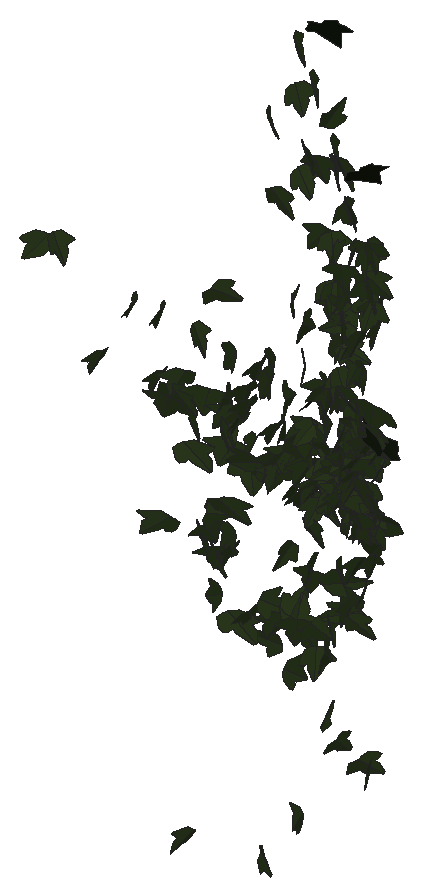
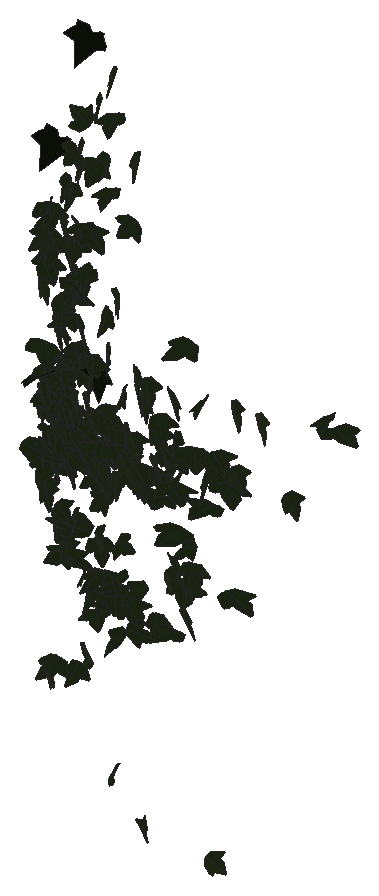
# SketchUp Ruby script. Lengths in millimetres.
U = 1.mm
M = Sketchup.active_model
def pt(a) = Geom::Point3d.new(a.map { |v| v * U })
def face(e, loops, mat)
  f = e.add_face(loops[0].map { |a| pt(a) })
  loops[1..].each { |l| e.add_face(l.map { |a| pt(a) }).erase! }
  f.material = f.back_material = mat if mat
  f
end
# faces: each face lists its corners as indices into pts; further lists are holes
def faces(e, pts, list, mat = nil) = list.each { |f| face(e, (f[0].is_a?(Array) ? f : [f]).map { |l| l.map { |i| pts[i] } }, mat) }
# xy, xz, yz: faces in a plane at the given z, y or x. An outline is a flat list of corners, or four numbers for a rectangle; further outlines are holes
def ring(l) = l.size == 4 ? [[l[0], l[1]], [l[2], l[1]], [l[2], l[3]], [l[0], l[3]]] : l.each_slice(2).to_a
def flat(e, list, mat, &to3) = list.each { |f| face(e, (f[0].is_a?(Array) ? f : [f]).map { |l| ring(l).map { |u, v| to3.(u, v) } }, mat) }
def xy(e, z, list, mat = nil) = flat(e, list, mat) { |x, y| [x, y, z] }
def xz(e, y, list, mat = nil) = flat(e, list, mat) { |x, z| [x, y, z] }
def yz(e, x, list, mat = nil) = flat(e, list, mat) { |y, z| [x, y, z] }
def lines(e, pts, list) = list.each { |a, b| e.add_line(pt(pts[a]), pt(pts[b])) }
# prism: a flat outline (further loops are holes) pulled along v
def prism(e, loops, v, mat = nil)
  f = face(e, loops, mat); d = Geom::Vector3d.new(v.map { |x| x * U })
  f.pushpull(f.normal.samedirection?(d) ? d.length : -d.length)
end
def box(e, o, s, mat = nil) = prism(e, [[o, [o[0] + s[0], o[1], o[2]], [o[0] + s[0], o[1] + s[1], o[2]], [o[0], o[1] + s[1], o[2]]]], [0, 0, s[2]], mat)
def at(x, y, z, deg = 0) = Geom::Transformation.translation(pt([x, y, z])) * Geom::Transformation.rotation(ORIGIN, Z_AXIS, deg.degrees)
def axes(o, x, y, z) = Geom::Transformation.new([*x, 0, *y, 0, *z, 0, *pt(o).to_a, 1])
def part(name) = M.definitions.add(name)
# library, detail: a bought-in or finely detailed component or shape, given as its bounding box
def library(name, o, s) = part(name).tap { |d| box(d.entities, o, s) }
def detail(e, o, s) = box(e.add_group.entities, o, s)
def put(e, d, t, mat = nil) = e.add_instance(d, t).tap { |i| i.material = mat if mat }
def group(e, t, mat = nil) = e.add_group.tap { |g| g.transformation = t; g.material = mat if mat }.entities
root = M.entities
M.materials.add("efeu1").color = [18, 25, 13]
M.materials.add("efeu2").color = [43, 57, 29]
c1 = part("ivyleaf_10")
p = [[0,12.8,-0.8],[-1.5,51.3,-10.9],[-4.9,51,-11.6],[-13.6,26.5,-7.3],[-13.2,15.9,-4.6],[-21.1,19.3,-7.2],
  [-29.5,16.3,-8.3],[-29.2,8.3,-6.2],[-19.7,-9.8,0.5],[-7.6,-13,4],[1,-12.2,5.8],[-0.4,51.1,-11.1],
  [-1.5,51.1,-10.9],[1,-12.4,5.9],[16.9,-12.4,3.5],[35.1,9.1,-5.1],[35,12.9,-6.1],[20.5,16.4,-4.9],
  [15.8,15,-3.8],[15.3,27.6,-7.1],[12.8,31.3,-7.8]]
faces(c1.entities,p,[[0,1,2,3,4,5,6,7,8,9,10],[11,12,0,13,14,15,16,17,18,19,20]],"efeu2")
c2 = part("ivyleaf_9")
p = [[39.1,54.8,31.7],[34.5,51.8,30.2],[-5.3,25.2,17.3],[-17.9,28.3,20.9],[-21.6,21.7,17],[-20.2,4.3,5.3],
  [-22.9,-0.3,2.5],[-17.1,-4,-0.6],[-2,-2.1,-1.2],[-0.7,-15.4,-10.1],[16.6,-22.3,-16.7],[21.1,-15.1,-12.5],
  [32.7,-10.7,-11],[46.1,-1.8,-6.6],[30.8,11.2,3.8]]
faces(c2.entities,p,[[0,1,2,3,4,5,6,7,8,9,10,11,12,13,14]],"efeu1")
put(root,c1,axes([280.1,1052.8,968.5],[0.80432,0.38706,-0.36071],[-0.57294,-0.20372,-0.57131],[-0.82806,0.51692,0.04493]))
put(root,c1,axes([304.2,1049,979.4],[0.14498,0.67726,0.04064],[-0.0098,0.04147,-0.68146],[-1.29124,0.07573,0.00973]))
put(root,c1,axes([369.6,1059.6,820.7],[-0.10799,-0.6367,0.11101],[0.00127,-0.1115,-0.63914],[1.23005,-0.05578,0.01041]))
put(root,c1,axes([435.9,1048.1,929.1],[0.18821,-0.63502,-0.20371],[-0.07183,0.20028,-0.64264],[1.2672,0.10567,-0.00617]))
put(root,c1,axes([474.4,1058,828.7],[-0.07826,-0.64651,0.07347],[-0.00557,-0.07344,-0.64781],[1.23834,-0.04119,0.00173]))
put(root,c1,axes([485.9,1053.1,609.2],[-0.72644,-0.3296,0.38813],[-0.44742,-0.31621,-0.49971],[0.85963,-0.44311,0.0679]))
put(root,c1,axes([484.6,1047.2,933.6],[0.18486,-0.65896,-0.1229],[0.01618,0.12538,-0.66557],[1.27566,0.0939,0.02625]))
put(root,c1,axes([496.1,1051,796.7],[-1.17512,-0.07231,0.17501],[-0.33467,-0.00247,-0.62142],[0.13369,-0.64176,-0.01733]))
put(root,c1,axes([514.7,1056,841],[-0.50585,-0.5574,0.22476],[-0.00833,-0.24396,-0.61018],[1.14381,-0.24829,0.09496]))
put(root,c1,axes([507.6,1049.3,818.6],[-1.10365,0.06979,-0.28827],[0.53343,-0.07811,-0.58274],[-0.18462,-0.64286,0.03951]))
put(root,c1,axes([524.9,1054.5,138.6],[-0.02119,-0.50512,0.39183],[-0.00233,-0.39187,-0.50521],[1.21668,-0.00955,0.00586]))
put(root,c1,axes([543.1,1043.6,782.1],[-0.43934,0.51009,0.32121],[-0.30419,0.27986,-0.55928],[-1.10619,-0.27955,0.02622]))
put(root,c1,axes([546,1048.1,923.3],[-0.06976,0.6764,0.00446],[-0.00032,0.00445,-0.67739],[-1.28735,-0.03666,-0.00007]))
put(root,c1,axes([537.8,1041.8,741.6],[0.76421,0.35078,0.36417],[0.45923,0.27573,-0.53165],[-0.84568,0.46672,0.04039]))
put(root,c1,axes([561.3,1049.4,597.1],[-0.64382,0.54486,-0.11963],[-0.12189,0.10105,0.64133],[1.05466,0.34429,0.00109]))
put(root,c1,axes([561.7,1053.1,830.7],[-1.06464,-0.33047,0.09999],[-0.02614,-0.16892,-0.63514],[0.65658,-0.54257,0.13684]))
put(root,c1,axes([565.4,1050,628.1],[-0.52647,-0.55222,-0.22368],[0.22261,0.19147,-0.61738],[1.11186,-0.29982,0.0177]))
put(root,c1,axes([579.5,1053.7,594.6],[-0.80133,-0.49881,-0.03379],[0.04217,0.02551,-0.65276],[0.95058,-0.42162,0.00047]))
put(root,c1,axes([585.6,1042.1,535],[0.38899,-0.41925,-0.46224],[-0.40776,0.4097,-0.46633],[1.1155,0.29596,-0.00927]))
put(root,c1,axes([576.9,1038.2,658.1],[-0.0198,-0.29068,-0.5946],[0.48061,0.54794,-0.27229],[1.16433,-0.23112,0.10228]))
put(root,c1,axes([568,1056.1,585.7],[0.19112,-0.21579,0.59118],[0.95073,-0.33678,-0.20779],[0.72848,0.49614,0.11608]))
put(root,c1,axes([584.2,1058,786.8],[-0.13485,0.63887,-0.1144],[0.00021,-0.11507,-0.64267],[-1.23525,-0.06977,0.01238]))
put(root,c1,axes([598.3,1057.9,760.7],[-0.98695,-0.29802,0.24077],[-0.1698,-0.30011,-0.56363],[0.70911,-0.48665,0.20014]))
put(root,c1,axes([585,1040.5,1003.5],[-0.47824,-0.34217,-0.55231],[0.64589,0.43584,-0.42442],[1.05443,-0.42217,0.00948]))
put(root,c1,axes([604.9,1055.4,816.3],[-0.64473,-0.45424,0.33849],[-0.32581,-0.29387,-0.56569],[1.02774,-0.37812,0.03301]))
put(root,c1,axes([596.4,1048.6,843.9],[0.13324,-0.56152,-0.34486],[0.16327,0.35162,-0.55511],[1.24347,0.014,0.10984]))
put(root,c1,axes([592.7,1056.8,798.1],[0.04256,0.65463,-0.0365],[-0.00251,-0.03648,-0.65501],[-1.24782,0.0224,0.00007]))
put(root,c1,axes([600.8,1051.3,629],[0.72732,-0.48918,-0.19687],[-0.14187,0.19057,-0.61824],[0.99349,0.38533,0.05584]))
put(root,c1,axes([601.7,1057.8,605.7],[0.10367,-0.62598,0.15616],[0.00987,-0.15628,-0.6283],[1.22784,0.05411,-0.00814]))
put(root,c1,axes([608.1,1045.3,911.5],[0.65528,-0.54496,-0.20928],[-0.10038,0.21293,-0.64125],[1.10647,0.34206,0.06577]))
put(root,c1,axes([596.7,1044.7,677.7],[-1.03918,-0.15423,-0.35911],[0.64836,0.11457,-0.56718],[0.36455,-0.6434,-0.01491]))
put(root,c1,axes([610,1055.9,808.4],[0.22548,-0.64019,-0.09152],[-0.00084,0.09296,-0.65086],[1.2308,0.11734,0.01632]))
put(root,c1,axes([627.8,1050.1,862.8],[-0.37925,-0.6345,-0.1009],[0.02524,0.10155,-0.66482],[1.22249,-0.19893,-0.01758]))
put(root,c1,axes([609.4,1047.8,502.6],[0.85017,0.33533,0.35778],[0.55087,0.21036,-0.55854],[-0.75333,0.53226,-0.00466]))
put(root,c1,axes([629.5,1052.7,840.4],[-0.24515,-0.65142,-0.05506],[0.01019,0.05506,-0.66401],[1.24416,-0.12881,-0.00541]))
put(root,c1,axes([632.8,1051.8,517.3],[-0.31182,-0.56641,-0.24556],[0.10948,0.23895,-0.58954],[1.16983,-0.17334,-0.01028]))
put(root,c1,axes([646.4,1042.4,758.3],[0.77283,-0.02268,-0.50401],[-0.84507,0.29111,-0.37084],[0.45589,0.57807,0.16698]))
put(root,c1,axes([638.8,1049.9,784.5],[0.53287,-0.61772,0.01758],[0.01416,-0.01592,-0.67821],[1.17604,0.28008,0.0002]))
put(root,c1,axes([628.3,1056.6,736.7],[1.22814,-0.01167,0.17544],[0.33338,-0.01503,-0.64531],[0.02894,0.66856,-0.01145]))
put(root,c1,axes([655.6,1045.1,912.8],[-0.08785,-0.67224,-0.12382],[0.02034,0.12338,-0.67382],[1.30076,-0.04733,0.00217]))
put(root,c1,axes([660.1,1060.3,750.3],[-0.13337,-0.64013,0.02762],[0.00929,-0.02831,-0.64391],[1.21939,-0.0698,0.00792]))
put(root,c1,axes([673.4,1055.6,485],[0.03445,0.03695,-0.70207],[-0.82529,0.19278,-0.01706],[0.23358,0.67567,0.04326]))
put(root,c1,axes([665.2,1057.9,765.8],[-0.23005,-0.60941,0.17977],[-0.08482,-0.17441,-0.62121],[1.20627,-0.12849,-0.0094]))
put(root,c1,axes([662.6,1048.3,887],[0.7927,-0.51225,-0.15366],[0.01192,0.19942,-0.64783],[1.01775,0.39664,0.12727]))
put(root,c1,axes([649.6,1057.6,145.3],[0.04948,-0.02956,0.63621],[0.9191,-0.41422,-0.03898],[0.79027,0.48359,0.0055]))
put(root,c1,axes([673.5,1056.8,817.2],[-0.11354,-0.65426,-0.02118],[-0.01753,0.0221,-0.65688],[1.24572,-0.05932,-0.01117]))
put(root,c1,axes([672.6,1047,896.4],[0.51298,-0.59828,-0.18198],[-0.00743,0.19655,-0.65196],[1.19013,0.2591,0.07437]))
put(root,c1,axes([678.4,1041.6,1296.1],[-0.54273,0.42017,0.38541],[-0.32115,0.28226,-0.61157],[-0.61702,-0.5165,-0.02069]))
put(root,c1,axes([670.4,1041.8,552],[0.08884,0.38468,0.60598],[0.10993,0.59937,-0.39131],[-0.86874,0.11518,0.01245]))
put(root,c1,axes([683.2,1056.8,525],[-0.56316,-0.56367,0.2269],[-0.14207,-0.21674,-0.63577],[1.14767,-0.30342,0.03264]))
put(root,c1,axes([677.4,1044.8,925.6],[0.58022,-0.55116,-0.27285],[0.00028,0.30461,-0.61513],[1.17046,0.27314,0.13541]))
put(root,c1,axes([682.2,1044.2,748],[0.35069,-0.59688,-0.22796],[-0.0606,0.22837,-0.62371],[1.2145,0.18375,0.0347]))
put(root,c1,axes([684.4,1055.7,752.9],[-0.54362,-0.52681,0.236],[-0.03889,-0.25391,-0.59154],[1.09794,-0.26983,0.0959]))
put(root,c1,axes([687.5,1060.9,776.1],[-0.09249,-0.63599,0.10402],[-0.03026,-0.1031,-0.6378],[1.22613,-0.05052,-0.00789]))
put(root,c1,axes([682.1,1049.1,1181.9],[-0.71162,0.11038,-0.40021],[0.46362,-0.13593,-0.59136],[-0.20393,-0.69421,0.05216]))
put(root,c1,axes([693.1,1063.7,632.4],[0.05493,0.48939,-0.48758],[-0.3037,-0.4443,-0.46893],[-0.78618,0.20582,0.14708]))
put(root,c1,axes([690.8,1052.1,826.1],[0.33863,-0.574,-0.2759],[0.09951,0.29867,-0.58764],[1.20799,0.1363,0.12575]))
put(root,c1,axes([703.5,1057.6,786.3],[-0.94893,-0.37717,0.18792],[-0.11506,-0.22408,-0.61017],[0.7937,-0.48343,0.13621]))
put(root,c1,axes([704.5,1040.5,878.4],[0.17993,-0.25751,-0.64935],[0.0939,0.6561,-0.253],[1.32615,-0.01152,0.10602]))
put(root,c1,axes([707.4,1056.4,737.8],[0.01575,-0.59983,-0.22154],[0.06168,0.22167,-0.59896],[1.21541,-0.00348,0.03327]))
put(root,c1,axes([710.2,1042.6,458.7],[-0.03949,0.42903,0.62238],[-0.11634,0.61565,-0.42935],[-0.91486,-0.09681,0.02773]))
put(root,c1,axes([723.9,1033.1,1033.5],[0.02742,0.1723,0.69331],[-0.78872,0.56687,-0.13226],[-1.10751,-0.39944,0.11136]))
put(root,c1,axes([708.3,1064.8,223.8],[-0.24162,0.01373,0.63664],[0.53678,-0.58081,0.06877],[1.08657,0.28998,0.10759]))
put(root,c1,axes([718.1,1056.9,730.5],[-0.15989,-0.60914,-0.1781],[0.04975,0.17618,-0.6149],[1.20682,-0.08797,0.00175]))
put(root,c1,axes([711,1047.6,552.6],[0.32929,0.4724,-0.5018],[0.29847,0.43814,0.54406],[0.78604,-0.36427,0.00363]))
put(root,c1,axes([720.9,1046.9,533.2],[-0.70789,-0.4564,0.07783],[-0.08124,-0.04122,-0.73818],[0.55898,-0.58398,-0.00872]))
put(root,c1,axes([712.9,1050.7,536.4],[0.7773,0.3037,-0.20744],[0.22867,0.08888,0.70581],[0.38605,-0.66413,-0.00041]))
put(root,c1,axes([720.2,1047.1,1428.5],[-0.42691,0.64337,0.15248],[-0.10326,0.12751,-0.73226],[-0.80002,-0.35978,0.01314]))
put(root,c1,axes([718.4,1048.4,1353.8],[0.39427,0.63237,0.11758],[0.00984,0.12759,-0.70839],[-0.78465,0.31935,0.0502]))
put(root,c1,axes([726.6,1054,825.7],[-0.28175,-0.64309,-0.06517],[0.0151,0.06505,-0.65987],[1.2301,-0.14809,-0.00683]))
put(root,c1,axes([734.6,1056.5,838.5],[-0.35471,-0.34286,0.56571],[-0.45682,-0.42411,-0.44949],[0.66529,-0.47402,-0.00702]))
put(root,c1,axes([730,1054.8,782.5],[-0.38704,-0.59074,0.1892],[-0.0308,-0.19399,-0.62308],[1.18015,-0.1988,0.04579]))
put(root,c1,axes([722.6,1044.6,808.6],[-0.86242,-0.0504,-0.23627],[0.28807,0.01034,-0.70867],[0.06232,-0.74527,0.00614]))
put(root,c1,axes([731,1051.8,778.2],[-0.36019,-0.59193,0.19072],[-0.04387,-0.19254,-0.62046],[1.18278,-0.1874,0.03507]))
put(root,c1,axes([722.6,1051.7,1224.9],[0.29001,0.63936,0.18485],[0.09862,0.16709,-0.68191],[-0.80595,0.25051,-0.01693]))
put(root,c1,axes([736.4,1039.2,940],[0.26272,-0.37261,-0.62387],[-0.20626,0.60714,-0.42098],[0.86221,0.25878,0.08939]))
put(root,c1,axes([734,1053.5,809.9],[0.56083,-0.58013,-0.09412],[-0.04865,0.09253,-0.6504],[1.11748,0.29518,0.01892]))
put(root,c1,axes([739.4,1055.7,613],[-0.77622,-0.16491,0.17004],[-0.20012,-0.04484,-0.65727],[0.20848,-0.65705,0.00218]))
put(root,c1,axes([734.6,1049.1,522.3],[-0.62799,-0.34601,-0.14546],[0.14847,0.0797,-0.62023],[0.43318,-0.52893,0.0017]))
put(root,c1,axes([739.2,1053.1,841.6],[0.50488,0.34265,-0.39183],[-0.36844,-0.24965,-0.53728],[-0.51722,0.51231,0.00025]))
put(root,c1,axes([736.8,1040.1,1004],[0.00355,-0.44298,-0.59748],[0.04866,0.59672,-0.44222],[0.90611,-0.03031,0.02609]))
put(root,c1,axes([734.3,1064.4,630.5],[0.30211,-0.54842,0.35009],[0.20014,-0.30985,-0.60144],[0.76813,0.29643,0.01901]))
put(root,c1,axes([740.8,1061.1,751.4],[-0.13094,-0.63941,0.05428],[-0.00526,-0.05429,-0.64309],[1.22129,-0.06879,0.00305]))
put(root,c1,axes([739.8,1058.6,750.8],[-0.13978,-0.5592,0.29973],[0.05125,-0.30421,-0.56096],[1.20643,-0.05187,0.05856]))
put(root,c1,axes([738.1,1043.2,1270.3],[-0.6488,0.49186,-0.02565],[0.0257,-0.015,-0.72439],[-0.60034,-0.53221,-0.00329]))
put(root,c1,axes([735.4,1054.4,690],[-0.60101,0.25831,-0.34202],[0.37315,-0.15315,-0.55622],[-0.36631,-0.57983,-0.00546]))
put(root,c1,axes([741.4,1054.2,1375.5],[-0.40851,0.64099,-0.09276],[0.00286,-0.10322,-0.72176],[-0.79015,-0.33177,0.04534]))
put(root,c1,axes([759.2,1052.2,824.2],[-0.36195,0.03985,0.59004],[-0.71403,0.07487,-0.29934],[-0.10345,-0.65617,0.00168]))
put(root,c1,axes([748.3,1055.5,723.2],[0.52253,0.49079,-0.25962],[-0.32433,-0.10659,-0.64007],[-0.59469,0.48937,0.12095]))
put(root,c1,axes([744.2,1055.6,492.2],[0.46112,0.62121,-0.07646],[-0.07922,-0.04992,-0.72657],[-0.75948,0.38238,0.02936]))
put(root,c1,axes([758,1057.5,1145.3],[-0.58993,-0.33267,0.38508],[-0.37938,-0.22731,-0.58686],[0.49142,-0.57483,0.00921]))
put(root,c2,axes([760.7,1035.6,899.2],[-0.00587,0.73457,0.24139],[-0.1084,0.23927,-0.72989],[-0.93707,-0.03228,0.08292]))
put(root,c1,axes([754.9,1047.5,1259.2],[-0.84142,-0.11486,-0.10799],[0.12842,0.02523,-0.69914],[0.14318,-0.69763,-0.00751]))
put(root,c1,axes([759,1051.4,886.7],[-0.41703,0.60905,0.1312],[-0.13926,0.08589,-0.69612],[-0.74722,-0.35592,0.05651]))
put(root,c1,axes([763.5,1050.1,914.7],[-0.74307,-0.40011,0.07551],[-0.03063,-0.0987,-0.72552],[0.4958,-0.60575,0.06834]))
put(root,c1,axes([770.9,1063.3,798.6],[-0.46788,-0.23761,0.5026],[-0.36873,-0.42336,-0.43077],[0.56926,-0.46952,0.13407]))
put(root,c1,axes([755.2,1039.1,545.3],[-0.38195,-0.48468,-0.46335],[0.53588,0.37804,-0.51739],[1.15819,-0.33475,0.08659]))
put(root,c1,axes([771.2,1045.9,916.2],[0.42523,-0.36414,-0.55987],[-0.31702,0.50783,-0.49206],[0.75061,0.42077,0.10935]))
put(root,c1,axes([766.7,1043.2,913.9],[-0.22812,-0.67729,-0.21292],[0.05119,0.20925,-0.70248],[0.86465,-0.19107,-0.01459]))
put(root,c1,axes([766.8,1053.8,850.7],[0.49008,-0.59026,-0.16503],[0.0047,0.18,-0.63996],[1.16645,0.24727,0.07191]))
put(root,c1,axes([762,1058.9,775.2],[1.03244,0.35695,-0.02191],[-0.03691,-0.01038,-0.64938],[-0.67963,0.54282,0.00199]))
put(root,c1,axes([768.9,1055.9,901.4],[-0.06,-0.68772,0.24142],[0.07686,-0.24508,-0.68529],[0.88589,-0.02532,0.07581]))
put(root,c1,axes([771.8,1040.4,508],[0.14065,-0.50236,-0.55334],[0.00914,0.56063,-0.50742],[0.91173,0.07188,0.09045]))
put(root,c1,axes([765.2,1057.8,762.4],[-1.07416,0.18765,-0.23674],[0.35067,-0.18371,-0.5849],[-0.45561,-0.58382,0.10796]))
put(root,c1,axes([768.1,1046.4,397.9],[0.51183,-0.56118,0.14321],[-0.11257,0.13045,0.62229],[-1.09651,-0.27534,0.00296]))
put(root,c1,axes([778.1,1063,752.6],[-0.26766,-0.41537,0.46283],[-0.13204,-0.46107,-0.43487],[1.17618,-0.14629,0.05651]))
put(root,c1,axes([781.7,1055.7,791.7],[0.2926,0.24368,-0.61379],[-0.61825,-0.3508,-0.33729],[-0.5166,0.55785,0.05601]))
put(root,c1,axes([768.8,1048.5,1065.6],[0.30232,0.62315,0.07576],[0.03339,0.07065,-0.67062],[-0.76512,0.24931,0.00067]))
put(root,c1,axes([775.5,1054.4,762.8],[0.45695,-0.60033,-0.06449],[-0.0295,0.06325,-0.6465],[1.14875,0.24043,0.00905]))
put(root,c2,axes([770.6,1038.5,1477.1],[0.72465,0.46252,-0.12405],[-0.09978,-0.09676,-0.75237],[-0.57563,0.59902,-0.02574]))
put(root,c1,axes([769.9,1055.3,551.7],[-0.23147,0.57199,-0.22008],[0.10225,-0.20401,-0.60246],[-0.74068,-0.20692,-0.01439]))
put(root,c1,axes([782,1054.5,984],[0.43738,-0.44174,-0.4577],[-0.33525,0.36628,-0.56875],[0.69989,0.4515,0.01359]))
put(root,c1,axes([755.8,1053.9,735.9],[0.52365,-0.17693,0.57143],[1.00572,-0.22289,-0.32345],[0.53356,0.59377,0.04886]))
put(root,c1,axes([771.2,1060.2,1257.1],[-0.4185,0.57342,-0.25785],[0.15052,-0.22662,-0.66812],[-0.75213,-0.36442,0.00976]))
put(root,c1,axes([774.8,1056.2,1286.9],[-0.41042,0.64415,-0.04422],[-0.01748,-0.0573,-0.72565],[-0.78752,-0.33443,0.03915]))
put(root,c1,axes([783.9,1056.8,791.9],[-0.45885,-0.60692,0.05726],[-0.06567,-0.04789,-0.6529],[1.15836,-0.24313,-0.01433]))
put(root,c1,axes([774.7,1071.3,820.4],[-0.04643,-0.05106,-0.69109],[0.05462,-0.69087,0.04858],[-0.84367,-0.04191,0.04118]))
put(root,c1,axes([775.7,1047,1326.6],[-0.09313,-0.65052,0.34299],[0.03292,0.34212,0.65488],[-0.89658,0.08013,-0.01158]))
put(root,c1,axes([776,1050.2,1145.1],[0.46505,0.55348,0.0293],[0.01953,0.02456,-0.67204],[-0.67591,0.38153,0.00075]))
put(root,c1,axes([788.6,1044.2,911.7],[-0.46759,0.54407,0.22852],[-0.41511,0.01888,-0.61563],[-0.58821,-0.44582,0.25281]))
put(root,c1,axes([779.6,1047.4,1068.7],[0.23362,0.62767,-0.13612],[-0.07614,-0.12319,-0.65581],[-0.77985,0.20006,0.02325]))
put(root,c1,axes([787.1,1048.1,1054.3],[-0.53942,-0.50523,0.15799],[-0.12707,-0.1188,-0.67137],[0.63319,-0.45425,-0.00014]))
put(root,c1,axes([786.1,1057.8,748.8],[-0.1284,-0.58687,0.25621],[0.0135,-0.25829,-0.58978],[1.21865,-0.05897,0.03353]))
put(root,c1,axes([792.1,1037.1,1130.2],[0.39412,0.00931,0.61207],[-0.58526,0.43375,0.24659],[-0.4639,-0.53931,0.2089]))
put(root,c1,axes([788.5,1050.7,915.6],[-0.83808,-0.16614,0.01577],[-0.01878,-0.00342,-0.70676],[0.20274,-0.68712,-0.0003]))
put(root,c1,axes([784.3,1054.2,929.9],[0.33263,0.57164,-0.16029],[-0.07054,-0.14998,-0.63322],[-0.72086,0.27845,-0.012]))
put(root,c1,axes([799.7,1051.3,1021.7],[0.33822,0.10228,-0.58345],[-0.69254,-0.13819,-0.29395],[-0.20648,0.63101,0.0302]))
put(root,c1,axes([803.8,1059.7,574.3],[0.75795,0.12397,-0.51768],[-0.96397,-0.11064,-0.41615],[-0.31167,0.6437,0.02817]))
put(root,c1,axes([787.8,1057.8,848.5],[0.40085,-0.56663,0.16094],[0.10927,-0.13409,-0.65493],[0.71028,0.34041,0.00993]))
put(root,c1,axes([793.8,1045.2,641.5],[-0.41165,0.41011,0.36563],[-0.28026,0.28446,-0.53107],[-0.60891,-0.40818,-0.00275]))
put(root,c1,axes([786.6,1053.6,938.5],[0.17346,0.62258,0.06943],[0.02006,0.06746,-0.6386],[-0.76399,0.14312,-0.001]))
put(root,c1,axes([795.3,1046.4,1064.6],[0.48574,-0.4127,-0.34597],[-0.26233,0.27265,-0.57269],[0.60237,0.45153,0.02958]))
put(root,c1,axes([788.8,1047.8,377.4],[-0.33195,-0.43726,-0.4379],[0.28119,0.41238,-0.47062],[1.14369,-0.2283,-0.01139]))
put(root,c1,axes([790.7,1051,1026.8],[-0.46682,0.47354,-0.26209],[0.15698,-0.23218,-0.60736],[-0.64137,-0.40149,0.0421]))
put(root,c1,axes([801.2,1052.7,1043.3],[0.68286,-0.02827,-0.35294],[-0.4301,0.0169,-0.56044],[0.04017,0.66149,-0.00077]))
put(root,c1,axes([799.1,1044.6,1108.4],[-0.76664,-0.25885,0.01291],[-0.01728,0.00048,-0.67959],[0.31572,-0.62852,-0.00584]))
put(root,c1,axes([793.5,1056.4,1025.5],[-0.14503,0.51849,-0.36064],[0.03924,-0.36152,-0.53037],[-0.76953,-0.11615,0.04092]))
put(root,c1,axes([799.1,1051.1,1075.7],[0.55406,-0.49626,-0.11124],[-0.09391,0.08034,-0.6727],[0.61332,0.46062,-0.00251]))
put(root,c1,axes([794.8,1059.5,789.7],[1.21149,-0.12359,-0.02219],[-0.01822,0.06655,-0.64533],[0.23828,0.63346,0.06347]))
put(root,c1,axes([791.9,1055,815.2],[0.25718,-0.47067,0.42743],[0.35397,-0.32947,-0.5059],[0.69019,0.34436,0.10019]))
put(root,c1,axes([795.3,1059.8,794.6],[0.70511,0.52121,-0.09834],[-0.10611,-0.08102,-0.63946],[-1.00387,0.37465,-0.00148]))
put(root,c1,axes([801.3,1058.3,587],[-0.00074,-0.65883,0.16871],[0.00544,-0.16871,-0.65881],[0.82969,0.00052,0.00447]))
put(root,c1,axes([783.9,1044.5,617.1],[-0.31698,-0.21523,0.6372],[0.70347,0.51913,0.27196],[-1.06939,0.40529,-0.00997]))
put(root,c1,axes([813.8,1053.9,885.2],[-0.26048,0.27092,-0.57718],[-0.63608,0.27619,0.3225],[0.44776,0.54995,0.12237]))
put(root,c1,axes([799,1047.8,1202.5],[-0.03337,-0.64301,-0.28223],[0.19933,0.26887,-0.6284],[0.83321,-0.09007,0.13903]))
put(root,c1,axes([803.4,1060.1,796.6],[-0.37155,-0.61364,0.05872],[0.07239,-0.07347,-0.64131],[1.17099,-0.19017,0.05828]))
put(root,c1,axes([811.6,1051.9,605.8],[-0.61564,-0.05558,0.38763],[-0.46582,-0.07059,-0.50717],[0.10611,-0.63239,0.02255]))
put(root,c1,axes([798.6,1062.6,736.5],[0.64329,-0.43545,0.13857],[0.11952,-0.09895,-0.68371],[0.54454,0.53614,-0.01364]))
put(root,c1,axes([796.9,1047.4,1269.2],[-0.68496,0.32969,-0.26763],[0.25513,-0.17147,-0.64993],[-0.4509,-0.59787,0.03882]))
put(root,c1,axes([804.5,1047.6,723.1],[0.57043,-0.5147,-0.24679],[-0.08754,0.25606,-0.58989],[1.08284,0.29184,0.08232]))
put(root,c1,axes([804,1052.8,808.1],[-0.80213,0.07766,-0.02077],[0.02775,0.01556,-0.66181],[-0.09407,-0.65763,-0.01811]))
put(root,c1,axes([788.3,1061.7,847.1],[0.01067,0.00964,-0.64829],[0.69619,-0.30789,0.00312],[-0.3755,-0.57057,-0.01263]))
put(root,c1,axes([806.3,1062,768.6],[-0.10896,-0.63325,0.0927],[-0.03241,-0.08985,-0.63937],[0.78013,-0.09218,-0.01362]))
put(root,c1,axes([803.1,1060.9,988.9],[-0.0778,0.18585,-0.61505],[-0.05046,-0.61798,-0.18245],[-0.78225,0.02138,0.07294]))
put(root,c1,axes([809.6,1050.4,822.8],[-0.84551,-0.48912,-0.03095],[0.0909,-0.00163,-0.65975],[0.92832,-0.44533,0.03641]))
put(root,c1,axes([810.7,1061.8,653.2],[-0.03845,-0.60197,0.25097],[-0.01952,-0.25048,-0.60279],[0.79544,-0.03524,-0.00266]))
put(root,c1,axes([797.9,1054.6,981.2],[-0.31582,-0.29696,-0.51076],[0.64932,0.12488,-0.34236],[0.31293,-0.55883,0.1949]))
put(root,c1,axes([811.6,1053.6,827.3],[0.55832,-0.54516,-0.20698],[-0.06324,0.21569,-0.6152],[1.108,0.28702,0.06918]))
put(root,c1,axes([812.8,1051.7,778.5],[-0.13435,-0.60616,0.23057],[0.04509,-0.23419,-0.60842],[1.23346,-0.05746,0.04735]))
put(root,c1,axes([819.8,1053,774.5],[-0.75949,-0.07937,0.30773],[-0.35447,-0.13208,-0.62184],[0.15709,-0.68176,0.08465]))
put(root,c1,axes([813.3,1055,957.6],[0.60765,-0.41094,-0.15334],[-0.14562,0.09628,-0.64571],[0.51492,0.51217,-0.00165]))
put(root,c1,axes([812.7,1052.9,1141.2],[0.39333,-0.60247,-0.07417],[-0.04447,0.06462,-0.68331],[0.73923,0.32445,-0.00164]))
put(root,c1,axes([814.9,1052.6,797.1],[0.00225,-0.65228,0.06383],[-0.01449,-0.06384,-0.65223],[1.24726,0.00043,-0.00769]))
put(root,c1,axes([811,1043.6,1208.5],[-0.60364,0.50117,-0.00216],[0.00168,-0.00168,-0.70426],[-0.61143,-0.49479,0.0002]))
put(root,c1,axes([816.2,1056.1,805.6],[0.26275,-0.58633,-0.24066],[-0.02276,0.24385,-0.60096],[1.20603,0.13234,0.04109]))
put(root,c1,axes([818.4,1053.7,812.4],[-1.03074,-0.36295,0.01386],[-0.02234,-0.00739,-0.65196],[0.69092,-0.54171,-0.00039]))
put(root,c1,axes([816.1,1058.3,1005.8],[-0.03379,-0.64316,0.16385],[-0.01848,-0.16334,-0.64371],[0.80951,-0.03058,-0.00785]))
put(root,c1,axes([818.7,1053.2,782],[-0.80514,0.25682,0.07306],[-0.0795,0.03401,-0.70812],[-0.31591,-0.66311,-0.00802]))
put(root,c1,axes([801.7,1052.7,832.9],[-0.17526,-0.00275,0.62823],[0.76254,0.06437,0.14321],[-0.0773,0.64122,-0.01169]))
put(root,c1,axes([816.2,1044.4,856.5],[0.12389,0.7108,0.20738],[-0.09665,0.21855,-0.71029],[-0.89814,0.07453,0.10504]))
put(root,c1,axes([819.3,1048.2,838.8],[0.45579,-0.63232,-0.08899],[-0.05967,0.07446,-0.73443],[0.77674,0.37676,-0.0042]))
put(root,c1,axes([821.6,1046.6,823.2],[-0.09805,-0.63412,-0.1975],[0.00901,0.19774,-0.63611],[1.264,-0.0506,-0.01079]))
put(root,c1,axes([803.6,1047.9,760.1],[0.31445,-0.08436,-0.62466],[0.76812,0.00193,0.25952],[-0.03706,-0.67575,0.07873]))
put(root,c1,axes([821.9,1042.7,726.8],[0.23769,-0.42232,-0.55143],[0.03369,0.57697,-0.43212],[0.8467,0.0956,0.172]))
put(root,c1,axes([813,1053,896.5],[0.68809,-0.2282,0.32278],[0.36615,-0.11881,-0.60842],[0.31387,0.63888,0.00215]))
put(root,c1,axes([812.8,1053,568.9],[-0.54581,-0.05685,-0.4497],[0.54933,0.01689,-0.45009],[0.06357,-0.63411,0.02833]))
put(root,c1,axes([811.3,1061.3,890.2],[0.19021,-0.22218,0.57986],[0.60404,-0.31636,-0.25434],[0.45724,0.51036,0.09478]))
put(root,c1,axes([820.3,1064,722],[0.50231,-0.49402,0.15947],[0.13886,-0.11267,-0.64293],[0.61791,0.42691,0.01485]))
put(root,c1,axes([819.6,1046.6,787.7],[-0.97777,0.36182,-0.17258],[0.25733,-0.10769,-0.6283],[-0.71823,-0.53115,0.00983]))
put(root,c1,axes([829.3,1053.4,839.3],[1.1141,0.16016,-0.26092],[-0.4853,-0.05654,-0.60678],[-0.32249,0.6384,0.01172]))
put(root,c1,axes([833.8,1055.5,744],[1.0379,0.11754,-0.33467],[-0.64076,-0.0217,-0.55624],[-0.21251,0.63948,0.04264]))
put(root,c1,axes([831.4,1046.3,959],[0.53579,-0.41036,-0.44287],[-0.2772,0.39505,-0.59137],[0.68244,0.48264,0.10749]))
put(root,c1,axes([831.6,1050,873.5],[-1.27981,0.05057,0.03675],[-0.0702,-0.00038,-0.67434],[-0.09606,-0.67345,0.00314]))
put(root,c1,axes([833.7,1053,853.4],[-0.43436,-0.61591,0.08269],[-0.07699,-0.07318,-0.65672],[1.18021,-0.23145,-0.01241]))
put(root,c1,axes([828.8,1045.9,735.2],[-0.82595,0.08676,-0.08449],[0.10104,-0.01835,-0.6825],[-0.10779,-0.68201,0.00762]))
put(root,c1,axes([833.2,1047.7,624.9],[0.20286,-0.57663,-0.35816],[-0.12791,0.3425,-0.60011],[0.81821,0.19651,-0.00501]))
put(root,c1,axes([835.3,1056.2,830.4],[-0.81132,-0.49666,0.00449],[0.0078,-0.00944,-0.65445],[0.94525,-0.42621,0.00926]))
put(root,c1,axes([834.8,1050.1,1094.3],[-0.32636,-0.66675,-0.19208],[0.20032,0.13918,-0.71182],[0.82248,-0.29847,0.09715]))
put(root,c2,axes([834,1038.8,1273.2],[0.53313,0.62088,0.10989],[0.06781,0.09525,-0.75919],[-0.76625,0.44041,0.00927]))
put(root,c1,axes([833.8,1061.2,774.7],[-0.70225,0.26008,-0.27985],[0.16824,-0.3305,-0.5908],[-0.43467,-0.5481,0.22345]))
put(root,c1,axes([840.3,1062.1,1061.9],[-0.08563,-0.6671,0.23811],[-0.01695,-0.23793,-0.6707],[0.86398,-0.07078,0.01044]))
put(root,c1,axes([840.4,1059.5,672.1],[-0.0301,-0.66145,0.00259],[-0.00043,-0.00258,-0.66191],[0.80697,-0.02468,-0.00026]))
put(root,c1,axes([842,1050,1154.3],[-0.79697,-0.33134,0.01624],[-0.02264,0.00068,-0.73242],[0.40408,-0.65345,-0.009]))
put(root,c1,axes([850.6,1049.7,866],[0.72867,-0.28571,-0.46144],[-0.59115,0.34773,-0.47303],[0.84705,0.48847,0.06683]))
put(root,c1,axes([841.6,1051.4,856.9],[0.15971,-0.63874,-0.13344],[0.02452,0.13613,-0.64354],[1.24166,0.07947,0.02987]))
put(root,c1,axes([838.4,1051,1143.9],[0.2333,0.70778,-0.10833],[-0.12421,-0.08411,-0.72926],[-0.86467,0.20305,0.07553]))
put(root,c1,axes([838.4,1056.1,355.2],[0.36509,-0.54013,0.29558],[0.21119,-0.24158,-0.61672],[0.72088,0.34433,0.03097]))
put(root,c1,axes([837.2,1039.8,366.5],[-0.5314,-0.41477,-0.49379],[0.53188,0.4071,-0.49998],[1.10608,-0.39503,0.00319]))
put(root,c1,axes([840.8,1052.5,715.3],[-0.77298,-0.4384,-0.2488],[0.36817,0.15949,-0.59682],[0.8859,-0.4488,0.03094]))
put(root,c1,axes([836.7,1061.6,676.5],[-0.67822,0.03531,0.40065],[0.47895,-0.10097,0.55362],[0.10669,0.67777,0.0616]))
put(root,c1,axes([843.6,1050,1063.2],[0.87707,0.11344,-0.10595],[-0.13922,0.04596,-0.72512],[-0.12837,0.72522,0.06253]))
put(root,c1,axes([842.2,1053,1092],[-0.16064,0.69238,-0.08177],[0.00693,-0.08215,-0.70472],[-0.85054,-0.13143,0.0097]))
put(root,c1,axes([845.4,1061.7,1029.6],[0.19588,-0.68096,0.10617],[0.06926,-0.09557,-0.69886],[0.83795,0.16708,0.03295]))
put(root,c1,axes([853.7,1046.4,909.3],[-1.25047,0.08671,0.13728],[-0.27351,-0.04418,-0.65989],[-0.14384,-0.66977,0.0613]))
put(root,c1,axes([850.3,1057.1,840.8],[0.25905,-0.63707,-0.0697],[-0.02426,0.06854,-0.65144],[1.21946,0.1367,0.00184]))
put(root,c1,axes([870.6,1056.9,735.3],[0.2428,0.19016,-0.60358],[-1.16952,0.18432,-0.07181],[0.28773,0.58873,0.21744]))
put(root,c1,axes([846.9,1046.8,1157.8],[-0.17208,0.7349,0.02508],[-0.03915,0.01936,-0.74779],[-0.89624,-0.14195,0.02785]))
put(root,c1,axes([848.3,1047.4,827],[-0.61327,-0.55138,-0.16214],[0.29435,0.09583,-0.63327],[1.05347,-0.34776,0.08256]))
put(root,c1,axes([843.1,1048.1,1108.6],[-0.67167,-0.22208,-0.45068],[0.52974,0.12605,-0.59254],[0.30839,-0.70023,0.03627]))
put(root,c1,axes([854.5,1056.7,819.4],[0.2477,-0.58817,-0.24812],[-0.03666,0.24949,-0.60153],[1.21438,0.1275,0.03245]))
put(root,c1,axes([854.7,1044.2,758.6],[0.558,-0.50509,-0.25376],[-0.02606,0.27943,-0.57201],[1.07546,0.26883,0.1178]))
put(root,c1,axes([857.2,1048.6,742.6],[0.3445,-0.48184,-0.40156],[-0.08277,0.4073,-0.50833],[1.19088,0.1677,0.08083]))
put(root,c2,axes([870.9,1041.3,856.2],[-0.15149,0.8107,0.01601],[-0.98115,-0.1252,0.10223],[0.12624,-0.00022,0.81375]))
